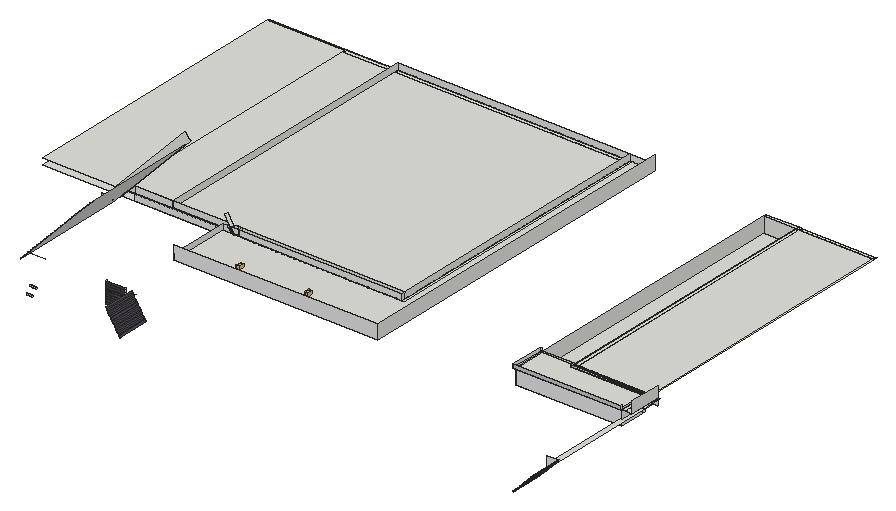
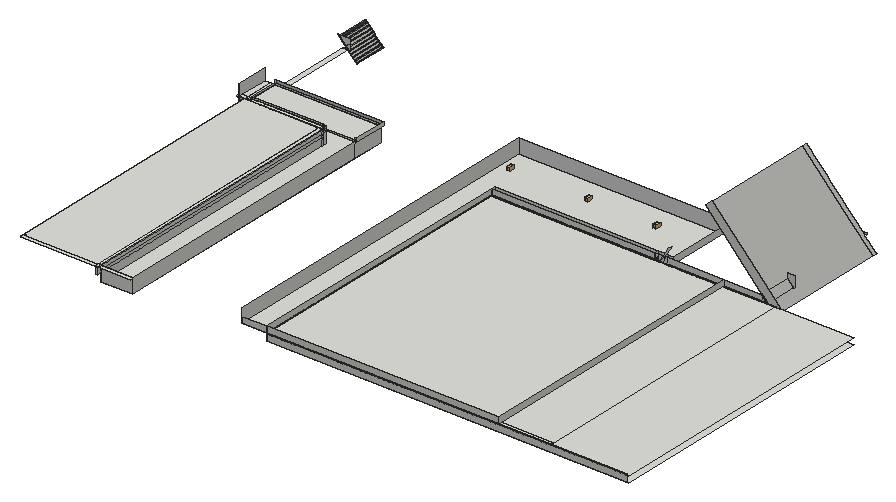
# SketchUp Ruby script. Lengths in inches.
U = 1.inch
M = Sketchup.active_model
def pt(a) = Geom::Point3d.new(a.map { |v| v * U })
def face(e, loops, mat)
  f = e.add_face(loops[0].map { |a| pt(a) })
  loops[1..].each { |l| e.add_face(l.map { |a| pt(a) }).erase! }
  f.material = f.back_material = mat if mat
  f
end
# faces: each face lists its corners as indices into pts; further lists are holes
def faces(e, pts, list, mat = nil) = list.each { |f| face(e, (f[0].is_a?(Array) ? f : [f]).map { |l| l.map { |i| pts[i] } }, mat) }
# xy, xz, yz: faces in a plane at the given z, y or x. An outline is a flat list of corners, or four numbers for a rectangle; further outlines are holes
def ring(l) = l.size == 4 ? [[l[0], l[1]], [l[2], l[1]], [l[2], l[3]], [l[0], l[3]]] : l.each_slice(2).to_a
def flat(e, list, mat, &to3) = list.each { |f| face(e, (f[0].is_a?(Array) ? f : [f]).map { |l| ring(l).map { |u, v| to3.(u, v) } }, mat) }
def xy(e, z, list, mat = nil) = flat(e, list, mat) { |x, y| [x, y, z] }
def xz(e, y, list, mat = nil) = flat(e, list, mat) { |x, z| [x, y, z] }
def yz(e, x, list, mat = nil) = flat(e, list, mat) { |y, z| [x, y, z] }
def lines(e, pts, list) = list.each { |a, b| e.add_line(pt(pts[a]), pt(pts[b])) }
# prism: a flat outline (further loops are holes) pulled along v
def prism(e, loops, v, mat = nil)
  f = face(e, loops, mat); d = Geom::Vector3d.new(v.map { |x| x * U })
  f.pushpull(f.normal.samedirection?(d) ? d.length : -d.length)
end
def box(e, o, s, mat = nil) = prism(e, [[o, [o[0] + s[0], o[1], o[2]], [o[0] + s[0], o[1] + s[1], o[2]], [o[0], o[1] + s[1], o[2]]]], [0, 0, s[2]], mat)
def at(x, y, z, deg = 0) = Geom::Transformation.translation(pt([x, y, z])) * Geom::Transformation.rotation(ORIGIN, Z_AXIS, deg.degrees)
def axes(o, x, y, z) = Geom::Transformation.new([*x, 0, *y, 0, *z, 0, *pt(o).to_a, 1])
def part(name) = M.definitions.add(name)
# library, detail: a bought-in or finely detailed component or shape, given as its bounding box
def library(name, o, s) = part(name).tap { |d| box(d.entities, o, s) }
def detail(e, o, s) = box(e.add_group.entities, o, s)
def put(e, d, t, mat = nil) = e.add_instance(d, t).tap { |i| i.material = mat if mat }
def group(e, t, mat = nil) = e.add_group.tap { |g| g.transformation = t; g.material = mat if mat }.entities
root = M.entities
M.materials.add("[Color M01]").color = [226, 226, 226]
M.materials.add("[Color M02]").color = [198, 198, 198]
M.materials.add("[Color M06]").color = [79, 71, 84]
c1 = library("Group\#13",[0,0,0],[3.54,3.54,3.9375])
xy(root,306.39,[[1464.52,523.75,1495.49,526.125]])
xy(root,307.2,[[1464.52,523.75,1495.49,526.125]])
xy(root,310.33,[[1464.52,523.75,1495.49,526.125]])
xy(root,311.14,[[1464.52,523.75,1495.49,526.125]])
xy(root,314.27,[[1464.52,523.75,1495.49,526.125]])
xy(root,315.08,[[1464.52,524.25,1495.49,526.125]])
xy(root,315.25,[[2025.57,678.64,2025.57,1195.68,2079.13,1195.68,2079.13,726.125,2202.51,726.125,2202.51,678.64]])
xy(root,318.2,[[1464.52,524.25,1495.49,526.125]])
xy(root,319.01,[[1464.52,524.25,1495.49,526.125]])
xy(root,322.14,[[1464.52,524.25,1495.49,526.125]])
xy(root,322.89,[[1464.52,524.25,1495.49,526.125]])
xy(root,326.02,[[1464.52,524.25,1495.49,526.125]])
xy(root,326.08,[[2200.93,528.48,2209.43,719.2],[2200.93,719.2,2209.43,719.59]])
xy(root,326.76,[[1464.52,524.25,1495.49,526.125]])
xy(root,328,[[1192.67,732.2,1797.03,1201.875]])
xy(root,329.89,[[1464.52,524.25,1495.49,526.125]])
xy(root,330.64,[[1464.52,524.25,1495.49,526.125]])
xy(root,333.125,[[2079.13,726.125,2082.95,732.2],[2079.13,732.2,2082.95,734.4375],[2079.13,734.4375,2082.95,1195.68]])
xy(root,333.77,[[1464.52,524.25,1495.49,526.125]])
xy(root,334.51,[[1464.52,524.25,1495.49,526.125]])
xy(root,336.02,[[2219.84,480.14,2220.09,480.77]])
xy(root,337.64,[[1464.52,524.25,1495.49,526.125]])
xy(root,338.39,[[1464.52,524.25,1495.49,526.125]])
xy(root,338.875,[[1192.67,732.2,1797.03,1201.875]])
xy(root,340.125,[[1497.82,623.84,1497.82,726.125,1550.15,726.125,1550.15,724.8125,1556.23,724.8125,1556.23,726.125,1559.65,726.125,1559.65,724.8125,1565.73,724.8125,1565.73,726.125,1569.15,726.125,1569.15,724.8125,1575.23,724.8125,1575.23,726.125,1578.65,726.125,1578.65,724.8125,1584.73,724.8125,1584.73,726.125,1588.15,726.125,1588.15,724.8125,1594.23,724.8125,1594.23,726.125,1597.65,726.125,1597.65,724.8125,1603.73,724.8125,1603.73,726.125,1607.15,726.125,1607.15,724.8125,1613.23,724.8125,1613.23,726.125,1616.65,726.125,1616.65,724.8125,1622.73,724.8125,1622.73,726.125,1626.15,726.125,1626.15,724.8125,1632.23,724.8125,1632.23,726.125,1635.65,726.125,1635.65,724.8125,1641.73,724.8125,1641.73,726.125,1645.15,726.125,1645.15,724.8125,1651.23,724.8125,1651.23,726.125,1654.65,726.125,1654.65,724.8125,1660.73,724.8125,1660.73,726.125,1664.15,726.125,1664.15,724.8125,1670.23,724.8125,1670.23,726.125,1673.65,726.125,1673.65,724.8125,1679.73,724.8125,1679.73,726.125,1683.15,726.125,1683.15,724.8125,1689.23,724.8125,1689.23,726.125,1692.65,726.125,1692.65,724.8125,1698.73,724.8125,1698.73,726.125,1702.15,726.125,1702.15,724.8125,1708.23,724.8125,1708.23,726.125,1711.65,726.125,1711.65,724.8125,1717.73,724.8125,1717.73,726.125,1721.15,726.125,1721.15,724.8125,1727.23,724.8125,1727.23,726.125,1730.65,726.125,1730.65,724.8125,1736.73,724.8125,1736.73,726.125,1740.15,726.125,1740.15,724.8125,1746.23,724.8125,1746.23,726.125,1749.65,726.125,1749.65,724.8125,1755.73,724.8125,1755.73,726.125,1759.15,726.125,1759.15,724.8125,1765.23,724.8125,1765.23,726.125,1768.65,726.125,1768.65,724.8125,1774.73,724.8125,1774.73,726.125,1778.15,726.125,1778.15,724.8125,1784.23,724.8125,1784.23,726.125,1787.65,726.125,1787.65,724.8125,1793.73,724.8125,1793.73,726.125,1797.15,726.125,1797.15,724.8125,1803.23,724.8125,1803.23,1201.875,1838.47,1201.875,1838.47,623.84],[2023.01,676.08,2025.57,678.64],[2025.57,676.08,2202.51,678.64],[2023.01,678.64,2025.57,732.2],[2025.57,678.64,2025.57,732.2,2079.13,732.2,2079.13,726.125,2202.51,726.125,2202.51,678.64],
  [2202.51,678.64,2208.71,726.125],[2208.71,678.64,2209.43,726.125],[2209.43,678.64,2219.8,726.125],[1550.15,724.8125,1556.23,726.125],[1559.65,724.8125,1565.73,726.125],
  [1569.15,724.8125,1575.23,726.125],[1578.65,724.8125,1584.73,726.125],[1588.15,724.8125,1594.23,726.125],[1597.65,724.8125,1603.73,726.125],[1607.15,724.8125,1613.23,726.125],
  [1616.65,724.8125,1622.73,726.125],[1626.15,724.8125,1632.23,726.125],[1635.65,724.8125,1641.73,726.125],[1645.15,724.8125,1651.23,726.125],[1654.65,724.8125,1660.73,726.125],
  [1664.15,724.8125,1670.23,726.125],[1673.65,724.8125,1679.73,726.125],[1683.15,724.8125,1689.23,726.125],[1692.65,724.8125,1698.73,726.125],[1702.15,724.8125,1708.23,726.125],
  [1711.65,724.8125,1717.73,726.125],[1721.15,724.8125,1727.23,726.125],[1730.65,724.8125,1736.73,726.125],[1740.15,724.8125,1746.23,726.125],[1749.65,724.8125,1755.73,726.125],
  [1759.15,724.8125,1765.23,726.125],[1768.65,724.8125,1774.73,726.125],[1778.15,724.8125,1784.23,726.125],[1787.65,724.8125,1793.73,726.125],[1797.15,724.8125,1803.23,1201.875],
  [1523.88,726.125,1797.03,732.2],[1797.03,726.125,1797.15,732.2],[2079.13,726.125,2085.21,732.2],[2085.21,726.125,2208.71,732.2],[2209.43,726.125,2219.8,732.2],
  [1322.96,732.2,1409.09,734.4375],[1409.09,732.2,1523.88,734.4375],[1523.88,732.2,1797.03,734.4375],[1797.03,732.2,1797.15,734.4375],[2079.13,732.2,2085.21,734.4375],
  [2085.21,732.2,2208.71,732.2,2208.71,732.32,2085.33,732.32,2085.33,734.4375,2085.21,734.4375],[2208.71,732.2,2209.43,734.4375],[2085.33,732.32,2208.71,734.4375],[1322.96,734.4375,1409.09,1195.68],[1409.09,734.4375,1797.03,1195.68],
  [1797.03,734.4375,1797.15,1195.8],[2079.13,734.4375,2085.21,1195.68],[2085.21,734.4375,2085.33,1195.68],[2085.33,734.4375,2208.71,1195.68],[2208.71,734.4375,2209.43,1195.68],
  [1322.96,1195.68,1409.09,1195.8],[1409.09,1195.68,1797.03,1195.8],[2025.57,1195.68,2079.13,1195.8],[2079.13,1195.68,2082.95,1195.8],[2082.95,1195.68,2085.21,1195.8],
  [2085.21,1195.68,2208.71,1195.8],[2208.71,1195.68,2209.43,1195.8],[1322.96,1195.8,1409.09,1201.875],[1409.09,1195.8,1797.03,1201.875],[1797.03,1195.8,1797.15,1201.875],
  [2025.57,1195.8,2079.13,1201.875],[2079.13,1195.8,2082.95,1201.875],[2082.95,1195.8,2085.21,1201.875],[2085.21,1195.8,2208.71,1201.875],[2208.71,1195.8,2209.43,1201.875]])
xz(root,480.64,[[1366.23,305.35,1368.54,307.67],[1369.14,305.35,1371.45,307.67],[1372.05,305.35,1374.36,307.67],[1374.96,305.35,1377.27,307.67]])
xz(root,480.7,[[1372.08,319.65,1374.39,321.96],[1374.99,319.65,1377.3,321.96],[1377.9,319.65,1380.22,321.96],[1380.81,319.65,1383.13,321.96]])
xz(root,521.5625,[[1532.53,305.32,1532.9,305.56,1531.21,308.2,1530.84,307.97],[2192,306.65,2191.54,307.08,2193.96,309.65,2194.42,309.22],[2191.54,307.08,2191.3125,307.29,2193.74,309.87,2193.96,309.65],[1530.31,308.8,1530.68,309.03,1528.98,311.68,1528.61,311.44],[2195.3,310.16,2194.84,310.59,2197.26,313.16,2197.72,312.73],
  [1528.08,312.27,1528.45,312.51,1526.75,315.15,1526.39,314.91],[2198.59,313.66,2198.14,314.09,2200.56,316.66,2201.02,316.23],[1525.85,315.74,1526.22,315.98,1524.53,318.62,1524.16,318.38],[2201.89,317.17,2201.4375,317.59,2202.51,318.73,2202.51,317.82],[2202.51,317.82,2202.96,318.3,2202.51,318.73],
  [2202.96,318.3,2204.3125,319.74,2203.86,320.17,2202.51,318.73],[2202.51,318.73,2203.86,320.17,2204.74,321.1,2207.16,323.67,2208.03,324.6,2209.43,326.08,2210.46,327.17,2211.33,328.11,2213.75,330.68,2214.63,331.61,2217.05,334.18,2217.93,335.11,2220.35,337.6875,2221.23,338.62,2222.65,340.125,2202.51,340.125],[1523.63,319.21,1524,319.45,1522.3,322.09,1521.93,321.86],[2205.19,320.67,2207.61,323.24,2207.16,323.67,2204.74,321.1],[1521.4,322.6875,1521.77,322.92,1520.08,325.57,1519.71,325.33],
  [2208.49,324.17,2208.03,324.6,2209.43,326.08,2209.43,325.17],[2209.43,325.17,2209.88,325.65,2209.43,326.08],[2209.88,325.65,2210.91,326.75,2210.46,327.17,2209.43,326.08],[1519.18,326.16,1519.54,326.4,1517.85,329.04,1517.48,328.8],[2211.79,327.68,2214.21,330.25,2213.75,330.68,2211.33,328.11],
  [1516.95,329.63,1517.32,329.87,1515.62,332.51,1515.25,332.28],[2215.09,331.18,2217.51,333.75,2217.05,334.18,2214.63,331.61],[1514.72,333.11,1515.09,333.34,1513.4,335.98,1513.03,335.75],[2218.39,334.6875,2220.81,337.26,2220.35,337.6875,2217.93,335.11],[1512.5,336.58,1512.86,336.8125,1511.17,339.46,1510.8,339.22],
  [1510.27,340.05,1510.64,340.29,1508.94,342.93,1508.58,342.69]])
xz(root,523.75,[[1464.52,307.2,1495.49,310.33],[1464.52,311.14,1495.49,314.27]],"[Color M06]")
xz(root,524.25,[[1464.52,315.08,1495.49,318.2],[1464.52,319.01,1495.49,322.14],[1464.52,322.89,1495.49,326.02],[1464.52,326.76,1495.49,329.89],[1464.52,330.64,1495.49,333.77],
  [1464.52,334.51,1495.49,337.64],[1464.52,338.39,1495.49,341.52]],"[Color M06]")
xz(root,526.125,[[1464.52,306.39,1495.49,307.2],[1464.52,310.33,1495.49,311.14],[1464.52,314.27,1495.49,315.08],[1464.52,318.2,1495.49,319.01],[1464.52,322.14,1495.49,322.89],
  [1464.52,326.02,1495.49,326.76],[1464.52,329.89,1495.49,330.64],[1464.52,333.77,1495.49,334.51],[1464.52,337.64,1495.49,338.39]])
xz(root,623.84,[[1497.82,340.125,1838.47,363.75]],"[Color M01]")
xz(root,676.08,[[2023.01,340.125,2202.51,346.3125]],"[Color M02]")
xz(root,678.64,[[1333.34,340.125,1336.18,340.125,1345.65,350.1875,1345.65,358.5,1333.34,358.5],[2025.57,340.125,2202.51,342.6875]])
xz(root,678.64,[[2025.57,315.25,2202.51,340.125]],"[Color M01]")
xz(root,726.125,[[2079.13,315.25,2082.95,333.125],[2082.95,315.25,2085.21,315.25,2085.21,340.125,2079.13,340.125,2079.13,333.125,2082.95,333.125],[2085.21,315.25,2197.32,340.125],[2197.32,315.25,2202.51,340.125],[1497.82,340.125,1497.82,350.1875,1504.29,350.1875,1510.74,340.125],
  [1510.74,340.125,1516.46,340.125,1510.01,350.1875,1504.29,350.1875],[1516.46,340.125,1510.01,350.1875,1523.88,350.1875,1523.88,340.125,1521.72,343.5],[1516.46,340.125,1521.72,343.5,1523.88,340.125],[1523.88,340.125,1797.03,350.1875],[2079.13,340.125,2085.21,342.6875],
  [2085.21,340.125,2197.32,342.6875],[2197.32,340.125,2202.51,342.6875]])
xz(root,731.75,[[1322.96,326.08,1312.29,336.13,1316.04,340.125,1332.61,357.73,1333.34,357.04,1333.34,358.5,1429.34,460.49,1436.88,453.39,1440.02,450.4375,1345.65,350.1875,1336.18,340.125]])
xz(root,732.2,[[2209.43,326.08,2209.43,328,2211.23,328],[1345.65,328,1504.29,338.875],[1504.29,328,1510.01,338.875],[1510.01,328,1517.43,328,1517.43,329.69,1511.54,338.875,1510.01,338.875],[1517.43,328,1518.52,328,1517.43,329.69],
  [1518.52,328,1523.88,328,1523.88,338.875,1517.43,338.875,1517.43,329.69],[1523.88,328,1797.03,338.875],[2079.13,328,2085.21,338.875],[2085.21,328,2209.43,338.875],[2209.43,328,2209.43,338.875,2219.8,338.875,2219.8,337.11,2211.23,328],
  [2211.23,328,2219.8,328,2219.8,337.11],[1517.43,329.69,1517.43,338.875,1511.54,338.875],[2219.8,337.11,2219.8,338.875,2221.47,338.875],[1335.01,338.875,1345.65,338.875,1345.65,340.125,1336.18,340.125],[1345.65,338.875,1504.29,340.125],
  [1504.29,338.875,1510.01,340.125],[1510.01,338.875,1511.54,338.875,1510.74,340.125,1510.01,340.125],[1511.54,338.875,1517.43,338.875,1517.43,340.125,1510.74,340.125],[1517.43,338.875,1523.88,340.125],[1523.88,338.875,1797.03,340.125],
  [2079.13,338.875,2085.21,340.125],[2085.21,338.875,2209.43,340.125],[2209.43,338.875,2219.8,340.125],[1336.18,340.125,1345.65,340.125,1345.65,350.1875],[1336.18,340.125,1345.65,350.1875,1409.09,350.1875,1409.09,340.125],
  [1345.65,340.125,1504.29,350.1875],[1504.29,340.125,1510.01,340.125,1510.01,341.27,1504.29,350.1875],[1510.01,340.125,1510.74,340.125,1510.01,341.27],[1510.74,340.125,1516.46,340.125,1510.01,350.1875,1510.01,341.27],[1516.46,340.125,1517.43,340.75,1517.43,350.1875,1510.01,350.1875],
  [1516.46,340.125,1517.43,340.125,1517.43,340.75],[1517.43,340.125,1523.88,340.125,1523.88,350.1875,1517.43,350.1875,1521.72,343.5,1517.43,340.75],[1523.88,340.125,1797.03,350.1875],[2023.01,340.125,2025.57,346.3125],[2025.57,340.125,2079.13,342.6875]])
xz(root,1195.68,[[2025.57,315.25,2079.13,340.125],[2079.13,333.125,2082.95,340.125]])
xz(root,1201.875,[[1196.48,328,1797.03,338.875],[2079.13,328,2082.95,338.875],[1196.48,338.875,1797.03,340.125],[2079.13,338.875,2082.95,340.125],[1409.09,340.125,1797.03,350.1875],
  [1797.03,340.125,1838.47,350.1875]])
yz(root,1409.09,[[732.2,340.125,1201.875,350.1875]])
yz(root,1464.52,[[523.75,307.2,526.125,310.33],[523.75,311.14,526.125,314.27],[524.25,315.08,526.125,318.2],[524.25,319.01,526.125,322.14],[524.25,322.89,526.125,326.02],
  [524.25,326.76,526.125,329.89],[524.25,330.64,526.125,333.77],[524.25,334.51,526.125,337.64],[524.25,338.39,526.125,341.52]])
yz(root,1495.49,[[523.75,307.2,526.125,310.33],[523.75,311.14,526.125,314.27],[524.25,315.08,526.125,318.2],[524.25,319.01,526.125,322.14],[524.25,322.89,526.125,326.02],
  [524.25,326.76,526.125,329.89],[524.25,330.64,526.125,333.77],[524.25,334.51,526.125,337.64],[524.25,338.39,526.125,341.52]])
yz(root,1497.82,[[623.84,340.125,726.125,350.1875]])
yz(root,1523.88,[[726.125,340.125,732.2,350.1875]])
yz(root,1797.03,[[732.2,328,1195.68,338.875],[1195.68,328,1201.875,338.875],[732.2,338.875,1195.68,340.125],[1195.68,338.875,1201.875,340.125],[726.125,340.125,732.2,350.1875],
  [732.2,340.125,1201.875,350.1875]])
yz(root,1838.47,[[623.84,340.125,1201.875,363.75]])
yz(root,2023.01,[[676.08,340.125,732.2,346.3125]])
yz(root,2025.57,[[678.64,315.25,732.2,340.125],[732.2,315.25,1195.68,340.125],[678.64,340.125,732.2,342.6875]])
yz(root,2079.13,[[726.125,315.25,732.2,333.125],[732.2,315.25,734.4375,328],[734.4375,315.25,1195.68,328],[732.2,328,734.4375,333.125],[734.4375,328,1195.68,333.125],
  [1195.68,328,1201.875,338.875],[726.125,333.125,732.2,340.125],[732.2,333.125,734.4375,338.875],[734.4375,333.125,1195.68,338.875],[732.2,338.875,734.4375,340.125],
  [734.4375,338.875,1195.68,340.125],[1195.68,338.875,1201.875,340.125],[726.125,340.125,732.2,342.6875]])
yz(root,2202.51,[[678.64,315.25,719.59,340.125],[719.59,315.25,726.125,340.125],[676.08,340.125,678.64,346.3125],[678.64,340.125,719.59,342.6875],[719.59,340.125,726.125,342.6875]])
yz(root,2209.43,[[726.125,326.08,732.2,340.125]])
yz(root,2219.8,[[678.64,340.125,731.75,358.5],[731.75,340.125,732.2,358.5]])
p = [[1530.84,521.5625,307.97],[1532.53,521.5625,305.32],[1532.53,467.1875,305.32],[1530.84,467.1875,307.97],[1532.9,521.5625,305.56],[1532.9,467.1875,305.56],
  [2190.66,521.5625,306.15],[2190.66,467.1875,306.15],[2191.12,467.1875,305.72],[2191.12,521.5625,305.72],[2190.4375,521.5625,306.36],[2190.4375,467.1875,306.36],
  [2191.54,521.5625,307.08],[2191.54,467.1875,307.08],[2192,521.5625,306.65],[2192,467.1875,306.65],[2194.42,521.5625,309.22],[2194.42,467.1875,309.22],
  [2191.3125,467.1875,307.29],[2191.3125,521.5625,307.29],[2193.96,521.5625,309.65],[2193.96,467.1875,309.65],[2193.74,521.5625,309.87],[2193.74,467.1875,309.87],
  [1531.21,467.1875,308.2],[1531.21,521.5625,308.2],[1530.68,467.1875,309.03],[1530.68,521.5625,309.03],[1528.61,521.5625,311.44],[1530.31,521.5625,308.8],
  [1530.31,467.1875,308.8],[1528.61,467.1875,311.44],[2194.84,521.5625,310.59],[2194.84,467.1875,310.59],[2195.3,521.5625,310.16],[2195.3,467.1875,310.16],
  [2197.72,521.5625,312.73],[2197.72,467.1875,312.73],[2197.26,521.5625,313.16],[2197.26,467.1875,313.16],[1528.98,467.1875,311.68],[1528.98,521.5625,311.68],
  [1528.45,467.1875,312.51],[1528.45,521.5625,312.51],[1526.39,521.5625,314.91],[1528.08,521.5625,312.27],[1528.08,467.1875,312.27],[1526.39,467.1875,314.91],
  [2198.14,521.5625,314.09],[2198.14,467.1875,314.09],[2198.59,521.5625,313.66],[2198.59,467.1875,313.66],[2201.02,521.5625,316.23],[2201.02,467.1875,316.23],
  [2200.56,521.5625,316.66],[2200.56,467.1875,316.66],[1526.75,467.1875,315.15],[1526.75,521.5625,315.15],[1526.22,467.1875,315.98],[1526.22,521.5625,315.98],
  [1524.16,521.5625,318.38],[1525.85,521.5625,315.74],[1525.85,467.1875,315.74],[1524.16,467.1875,318.38],[2201.4375,521.5625,317.59],[2201.4375,467.1875,317.59],
  [2201.89,521.5625,317.17],[2201.89,467.1875,317.17],[2202.96,521.5625,318.3],[2204.3125,521.5625,319.74],[2204.3125,467.1875,319.74],[2202.51,521.5625,317.82],
  [2203.86,521.5625,320.17],[2202.51,521.5625,318.73],[2203.86,467.1875,320.17],[1524.53,467.1875,318.62],[1524.53,521.5625,318.62],[1524,467.1875,319.45],
  [1524,521.5625,319.45],[1521.93,521.5625,321.86],[1523.63,521.5625,319.21],[1523.63,467.1875,319.21],[1521.93,467.1875,321.86],[2204.74,521.5625,321.1],
  [2204.74,467.1875,321.1],[2205.19,521.5625,320.67],[2205.19,467.1875,320.67],[2207.61,521.5625,323.24],[2207.61,467.1875,323.24],[2207.16,521.5625,323.67],
  [2207.16,467.1875,323.67],[1522.3,467.1875,322.09],[1522.3,521.5625,322.09],[1521.77,467.1875,322.92],[1521.77,521.5625,322.92],[1519.71,521.5625,325.33],
  [1521.4,521.5625,322.6875],[1521.4,467.1875,322.6875],[1519.71,467.1875,325.33],[2208.03,521.5625,324.6],[2208.03,467.1875,324.6],[2208.49,521.5625,324.17],
  [2208.49,467.1875,324.17],[2209.88,521.5625,325.65],[2210.91,521.5625,326.75],[2210.91,467.1875,326.75],[2209.43,521.5625,325.17],[2210.46,521.5625,327.17],
  [2209.43,521.5625,326.08],[2210.46,467.1875,327.17],[1520.08,467.1875,325.57],[1520.08,521.5625,325.57],[1519.54,467.1875,326.4],[1519.54,521.5625,326.4],
  [1322.96,528.48,326.08],[1440.02,528.48,450.4375],[1440.02,521.5625,450.4375],[1439.71,521.5625,450.11],[1439.44,521.5625,449.82],[1437.02,521.5625,447.25],
  [1436.14,521.5625,446.32],[1433.72,521.5625,443.75],[1432.84,521.5625,442.8125],[1430.42,521.5625,440.24],[1429.55,521.5625,439.31],[1427.125,521.5625,436.74],
  [1426.25,521.5625,435.81],[1423.83,521.5625,433.23],[1422.95,521.5625,432.3],[1420.53,521.5625,429.73],[1419.65,521.5625,428.8],[1417.23,521.5625,426.23],
  [1416.35,521.5625,425.29],[1413.93,521.5625,422.72],[1413.05,521.5625,421.79],[1410.63,521.5625,419.22],[1409.75,521.5625,418.28],[1407.33,521.5625,415.71],
  [1406.46,521.5625,414.78],[1404.03,521.5625,412.21],[1403.16,521.5625,411.28],[1400.74,521.5625,408.7],[1399.86,521.5625,407.77],[1397.4375,521.5625,405.2],
  [1396.56,521.5625,404.27],[1394.14,521.5625,401.7],[1393.26,521.5625,400.76],[1390.84,521.5625,398.19],[1389.96,521.5625,397.26],[1387.54,521.5625,394.6875],
  [1386.66,521.5625,393.75],[1384.24,521.5625,391.18],[1383.37,521.5625,390.25],[1380.94,521.5625,387.68],[1380.07,521.5625,386.75],[1377.65,521.5625,384.17],
  [1376.77,521.5625,383.24],[1374.35,521.5625,380.67],[1373.47,521.5625,379.74],[1371.05,521.5625,377.17],[1370.17,521.5625,376.23],[1367.75,521.5625,373.66],
  [1366.87,521.5625,372.73],[1364.45,521.5625,370.16],[1363.57,521.5625,369.23],[1361.15,521.5625,366.65],[1360.28,521.5625,365.72],[1357.85,521.5625,363.15],
  [1356.98,521.5625,362.22],[1354.56,521.5625,359.64],[1353.68,521.5625,358.71],[1351.26,521.5625,356.14],[1350.38,521.5625,355.21],[1347.96,521.5625,352.64],
  [1347.08,521.5625,351.7],[1344.66,521.5625,349.13],[1343.78,521.5625,348.2],[1341.36,521.5625,345.63],[1340.48,521.5625,344.7],[1338.0625,521.5625,342.125],
  [1337.1875,521.5625,341.19],[1336.18,521.5625,340.125],[1334.76,521.5625,338.62],[1333.89,521.5625,337.6875],[1331.47,521.5625,335.11],[1330.59,521.5625,334.18],
  [1328.17,521.5625,331.61],[1327.29,521.5625,330.68],[1324.87,521.5625,328.11],[1323.99,521.5625,327.17],[1322.96,521.5625,326.08],[1322.96,719.59,326.08],
  [1336.18,719.59,340.125],[1336.18,678.64,340.125],[1345.65,678.64,350.1875],[1345.65,719.59,350.1875],[1440.02,719.59,450.4375],[1322.96,719.2,326.08],
  [2209.43,719.59,326.08],[2209.43,719.2,326.08],[2198.75,719.2,336.13],[2198.75,731.75,336.13],[2209.43,731.75,326.08],[2209.43,726.125,326.08],
  [2222.65,719.59,340.125],[2222.65,726.125,340.125],[2222.65,731.75,340.125],[2222.65,732.2,340.125],[2221.47,732.2,338.875],[2219.8,732.2,337.11],
  [2211.23,732.2,328],[2209.43,732.2,326.08],[1517.48,521.5625,328.8],[1519.18,521.5625,326.16],[1519.18,467.1875,326.16],[1517.48,467.1875,328.8],
  [2211.33,521.5625,328.11],[2211.33,467.1875,328.11],[2211.79,521.5625,327.68],[2211.79,467.1875,327.68],[2214.21,521.5625,330.25],[2214.21,467.1875,330.25],
  [2213.75,521.5625,330.68],[2213.75,467.1875,330.68],[1517.85,467.1875,329.04],[1517.85,521.5625,329.04],[1517.32,467.1875,329.87],[1517.32,521.5625,329.87],
  [1515.25,521.5625,332.28],[1516.95,521.5625,329.63],[1516.95,467.1875,329.63],[1515.25,467.1875,332.28],[2214.63,521.5625,331.61],[2214.63,467.1875,331.61],
  [2215.09,521.5625,331.18],[2215.09,467.1875,331.18],[2217.51,521.5625,333.75],[2217.51,467.1875,333.75],[2217.05,521.5625,334.18],[2217.05,467.1875,334.18],
  [1515.62,467.1875,332.51],[1515.62,521.5625,332.51],[1515.09,467.1875,333.34],[1515.09,521.5625,333.34],[1513.03,521.5625,335.75],[1514.72,521.5625,333.11],
  [1514.72,467.1875,333.11],[1513.03,467.1875,335.75],[2219.84,480.14,336.02],[2217.77,480.14,333.82],[2217.77,480.77,333.82],[2219.84,480.77,336.02],
  [2217.93,521.5625,335.11],[2217.93,467.1875,335.11],[2218.39,521.5625,334.6875],[2218.39,467.1875,334.6875],[2220.81,521.5625,337.26],[2220.81,467.1875,337.26],
  [1513.4,467.1875,335.98],[1513.4,521.5625,335.98],[1512.86,467.1875,336.8125],[1512.86,521.5625,336.8125],[1510.8,521.5625,339.22],[1512.5,521.5625,336.58],
  [1512.5,467.1875,336.58],[1510.8,467.1875,339.22],[2220.35,521.5625,337.6875],[2220.35,467.1875,337.6875],[1511.17,467.1875,339.46],[1511.17,521.5625,339.46],
  [1510.64,467.1875,340.29],[1510.64,521.5625,340.29],[1510.74,521.5625,340.125],[1508.58,521.5625,342.69],[1510.27,521.5625,340.05],[1510.27,467.1875,340.05],
  [1508.58,467.1875,342.69],[1345.65,731.75,350.1875],[1336.18,731.75,340.125],[1336.18,726.125,340.125],[1501.3125,726.125,363.75],[1500.55,726.125,364.9375],
  [1500.55,732.2,364.9375],[1510.01,732.2,350.1875],[1516.46,732.2,340.125],[1516.46,726.125,340.125],[1510.01,726.125,350.1875],[1504.29,726.125,359.1],
  [1521.72,726.125,343.5],[1517.43,732.2,340.75],[1521.72,732.2,343.5],[1336.18,732.2,340.125],[1345.65,732.2,350.1875],[1365.01,521.5625,340.125],
  [1337.04,521.5625,340.125],[1516.46,521.5625,340.125],[2202.51,726.125,340.125],[2202.51,731.75,340.125],[2209.43,528.48,326.08],[2198.75,528.48,336.13]]
faces(root,p,[[0,1,2,3],[6,12,13,7],[13,12,14,15],[14,16,17,15],[24,26,27,25],[28,29,30,31],[20,32,33,21],[33,32,34,35],
  [34,36,37,35],[40,42,43,41],[44,45,46,47],[38,48,49,39],[50,52,53,51],[56,58,59,57],[60,61,62,63],[54,64,65,55],
  [68,69,70,67,66,71],[75,77,78,76],[79,80,81,82],[72,83,84,74],[85,87,88,86],[91,93,94,92],[95,96,97,98],[89,99,100,90],
  [103,104,105,102,101,106],[110,112,113,111],[212,213,214,215],[107,216,217,109],[218,220,221,219],[224,226,227,225],[228,229,230,231],[222,232,233,223],
  [234,236,237,235],[240,242,243,241],[244,245,246,247],[238,252,253,239],[254,256,257,255],[258,260,261,259],[262,263,264,265],[268,270,271,272,269],
  [273,274,275,276]],"[Color M06]")
faces(root,p,[[4,5,2,1],[6,7,8,9],[7,6,10,11],[12,13,18,19],[20,12,13,21],[22,19,18,23],[24,25,0,3],[27,26,30,29],
  [20,21,17,16],[21,20,22,23],[38,32,33,39],[40,41,28,31],[43,42,46,45],[38,39,37,36],[49,48,50,51],[54,48,49,55],
  [56,57,44,47],[59,58,62,61],[54,55,53,52],[65,64,66,67],[72,73,64,65,74],[75,76,60,63],[78,77,81,80],[72,74,70,69],
  [84,83,85,86],[89,83,84,90],[91,92,79,82],[94,93,97,96],[89,90,88,87],[100,99,101,102],[107,108,99,100,109],[110,111,95,98],
  [114,115,116,117,118,119,120,121,122,123,124,125,126,127,128,129,130,131,132,133,134,135,136,137,138,139,140,141,142,143,144,145,146,147,148,149,150,151,152,153,154,155,156,157,158,159,160,161,162,163,164,165,166,167,168,169,170,171,172,173,174,175,176,177,178,179,180,181,182,183,184,185,186,187,188,189,190],[191,192,193,194,195,196,115,114,197],[198,199,200,201,202,203],[198,204,205,206,202,203],[202,206,207,208,209,210,211],[113,112,214,213],[107,109,105,104],[217,216,218,219],
  [222,216,217,223],[224,225,212,215],[227,226,230,229],[222,223,221,220],[233,232,234,235],[238,232,233,239],[240,241,228,231],[243,242,246,245],
  [238,239,237,236],[248,249,250,251],[253,252,254,255],[258,259,244,247],[261,260,264,263],[266,267,257,256],[268,269,262,265],[271,270,275,274],
  [192,195,194,193],[192,195,277,278,279],[280,281,282,283,284,285,286,287],[288,285,284,289,290],[277,278,291,292]])
lines(root,p,[[293,294],[272,295],[296,297],[298,299]])
put(root,c1,axes([1579.86,658.52,344.6875],[-1.5535,0,0],[0,2.39,0],[0,0,-3.63878]))
put(root,c1,axes([1694.43,658.52,344.6875],[-1.5535,0,0],[0,2.39,0],[0,0,-3.63878]))
put(root,c1,axes([1824.99,658.52,344.6875],[-1.5535,0,0],[0,2.39,0],[0,0,-3.63878]))
